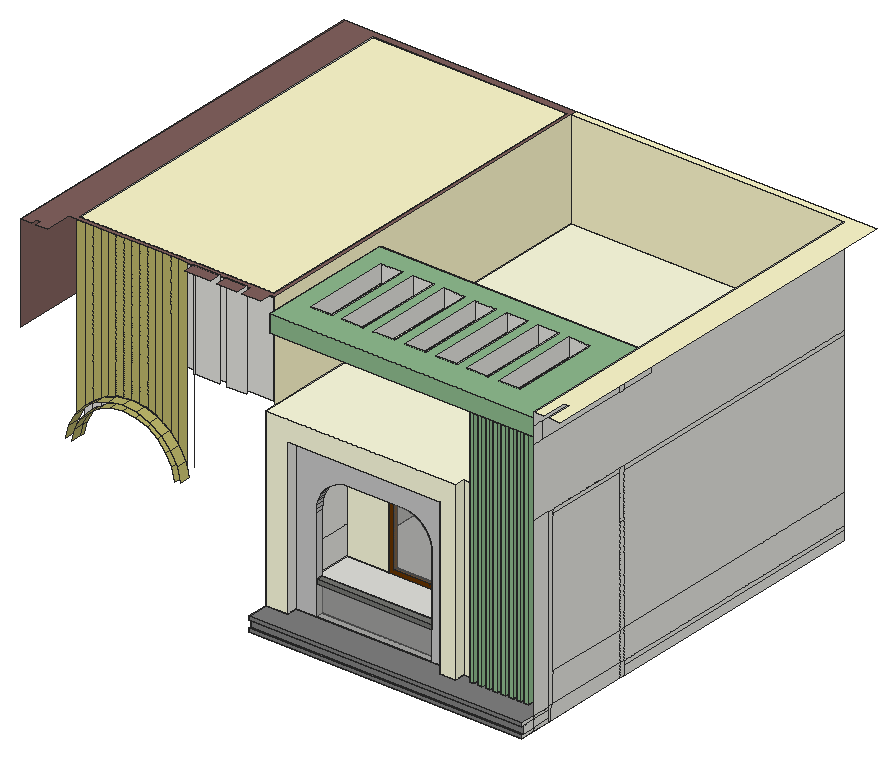
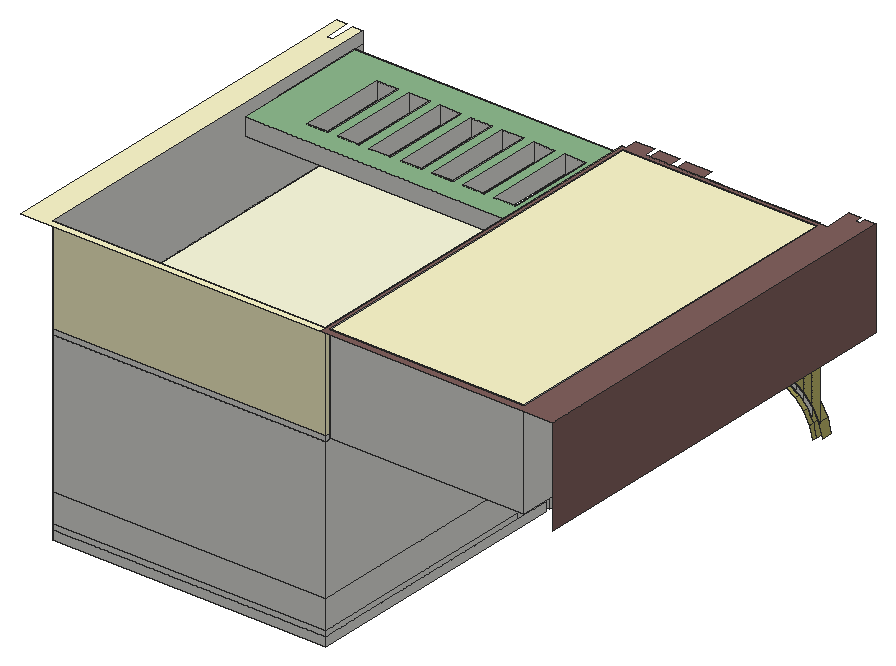
# SketchUp Ruby script. Lengths in inches.
U = 1.inch
M = Sketchup.active_model
def pt(a) = Geom::Point3d.new(a.map { |v| v * U })
def face(e, loops, mat)
  f = e.add_face(loops[0].map { |a| pt(a) })
  loops[1..].each { |l| e.add_face(l.map { |a| pt(a) }).erase! }
  f.material = f.back_material = mat if mat
  f
end
# faces: each face lists its corners as indices into pts; further lists are holes
def faces(e, pts, list, mat = nil) = list.each { |f| face(e, (f[0].is_a?(Array) ? f : [f]).map { |l| l.map { |i| pts[i] } }, mat) }
# xy, xz, yz: faces in a plane at the given z, y or x. An outline is a flat list of corners, or four numbers for a rectangle; further outlines are holes
def ring(l) = l.size == 4 ? [[l[0], l[1]], [l[2], l[1]], [l[2], l[3]], [l[0], l[3]]] : l.each_slice(2).to_a
def flat(e, list, mat, &to3) = list.each { |f| face(e, (f[0].is_a?(Array) ? f : [f]).map { |l| ring(l).map { |u, v| to3.(u, v) } }, mat) }
def xy(e, z, list, mat = nil) = flat(e, list, mat) { |x, y| [x, y, z] }
def xz(e, y, list, mat = nil) = flat(e, list, mat) { |x, z| [x, y, z] }
def yz(e, x, list, mat = nil) = flat(e, list, mat) { |y, z| [x, y, z] }
def lines(e, pts, list) = list.each { |a, b| e.add_line(pt(pts[a]), pt(pts[b])) }
# prism: a flat outline (further loops are holes) pulled along v
def prism(e, loops, v, mat = nil)
  f = face(e, loops, mat); d = Geom::Vector3d.new(v.map { |x| x * U })
  f.pushpull(f.normal.samedirection?(d) ? d.length : -d.length)
end
def box(e, o, s, mat = nil) = prism(e, [[o, [o[0] + s[0], o[1], o[2]], [o[0] + s[0], o[1] + s[1], o[2]], [o[0], o[1] + s[1], o[2]]]], [0, 0, s[2]], mat)
def at(x, y, z, deg = 0) = Geom::Transformation.translation(pt([x, y, z])) * Geom::Transformation.rotation(ORIGIN, Z_AXIS, deg.degrees)
def axes(o, x, y, z) = Geom::Transformation.new([*x, 0, *y, 0, *z, 0, *pt(o).to_a, 1])
def part(name) = M.definitions.add(name)
# library, detail: a bought-in or finely detailed component or shape, given as its bounding box
def library(name, o, s) = part(name).tap { |d| box(d.entities, o, s) }
def detail(e, o, s) = box(e.add_group.entities, o, s)
def put(e, d, t, mat = nil) = e.add_instance(d, t).tap { |i| i.material = mat if mat }
def group(e, t, mat = nil) = e.add_group.tap { |g| g.transformation = t; g.material = mat if mat }.entities
root = M.entities
M.materials.add("[0043_SaddleBrown]").color = [130, 97, 94]
M.materials.add("[0050_LemonChiffon]").color = [255, 250, 205]
M.materials.add("[0054_LightYellow]").color = [255, 255, 224]
M.materials.add("[0057_DarkKhaki]").color = [189, 183, 107]
M.materials.add("[0072_DarkSeaGreen]").color = [143, 188, 143]
M.materials.add("[0133_Gray]").color = [128, 128, 128]
M.materials.add("[Cladding Stucco White]").color = [200, 200, 200]
M.materials.add("[Color C08]").color = [102, 51, 0]
M.materials.add("[Color M00]").color = [255, 255, 255]
M.materials.add("[Metal Seamed]").color = [118, 119, 115]
M.materials.add("[Translucent Glass Gray]").color = [128, 128, 128]
M.materials["[Translucent Glass Gray]"].alpha = 0.5
M.materials.add("[Wood Floor Dark]").color = [153, 94, 42]
c1 = part("Group\#1")
xy(c1.entities,0,[[0,0,81.875,4.3125]],"[Color C08]")
xy(c1.entities,4.13,[[4.13,0,38.5,0.0625],[38.5,0,42.19,0.0625],[42.19,0,77.74,0.0625],[4.13,0.0625,38.5,4.3125],[38.5,0.0625,42.19,4.3125],
  [42.19,0.0625,77.74,4.3125]],"[Color C08]")
xy(c1.entities,128.34,[[4.13,0,38.5,0.0625],[42.19,0,77.74,0.0625],[4.13,0.0625,38.5,4.3125],[42.19,0.0625,77.74,4.3125]],"[Color C08]")
xy(c1.entities,132.48,[[0,0,81.875,4.3125]],"[Color C08]")
xz(c1.entities,0,[[[0,0,81.875,132.48],[4.13,4.13,4.13,128.34,38.5,128.34,38.5,4.13,42.19,4.13,42.19,128.34,77.74,128.34,77.74,4.13]]],"[Color C08]")
xz(c1.entities,0.0625,[[4.13,4.13,38.5,128.34],[42.19,4.13,77.74,128.34]],"[Translucent Glass Gray]")
xz(c1.entities,4.3125,[[[0,0,81.875,132.48],[4.13,4.13,77.74,4.13,77.74,128.34,42.19,128.34,42.19,4.13,38.5,4.13,38.5,128.34,4.13,128.34]]],"[Color C08]")
yz(c1.entities,0,[[0,0,4.3125,132.48]],"[Color C08]")
yz(c1.entities,4.13,[[0,4.13,0.0625,128.34],[0.0625,4.13,4.3125,128.34]],"[Color C08]")
yz(c1.entities,38.5,[[0,4.13,0.0625,128.34],[0.0625,4.13,4.3125,128.34]],"[Color C08]")
yz(c1.entities,42.19,[[0,4.13,0.0625,128.34],[0.0625,4.13,4.3125,128.34]],"[Color C08]")
yz(c1.entities,77.74,[[0,4.13,0.0625,128.34],[0.0625,4.13,4.3125,128.34]],"[Color C08]")
yz(c1.entities,81.875,[[0,0,4.3125,132.48]],"[Color C08]")
xy(root,302,[[287.625,134.125,287.625,173.6875,289.55,173.6875,289.55,167.4375,295.8,167.4375,295.8,173.6875,302.98,173.6875,302.98,167.4375,309.23,167.4375,309.23,173.6875,316.42,173.6875,316.42,167.4375,322.67,167.4375,322.67,173.6875,329.86,173.6875,329.86,167.4375,336.11,167.4375,336.11,173.6875,343.3,173.6875,343.3,167.4375,349.55,167.4375,349.55,173.6875,356.73,173.6875,356.73,167.4375,362.98,167.4375,362.98,173.6875,370.17,173.6875,370.17,167.4375,376.42,167.4375,376.42,173.6875,624.625,173.6875,624.625,134.125],[287.625,173.6875,624.625,285.75]],"[Wood Floor Dark]")
xy(root,306.0625,[[287.625,137,287.625,160.625,314.125,160.625,314.125,173.6875,502.3125,173.6875,502.3125,160.625,521.4375,160.625,521.4375,173.6875,534.24,173.6875,534.24,166.375,539.56,166.375,539.56,173.6875,544.06,173.6875,544.06,166.375,549.37,166.375,549.37,173.6875,553.87,173.6875,553.87,166.375,559.18,166.375,559.18,173.6875,563.68,173.6875,563.68,166.375,568.99,166.375,568.99,173.6875,573.49,173.6875,573.49,166.375,578.81,166.375,578.81,173.6875,583.31,173.6875,583.31,166.375,588.62,166.375,588.62,173.6875,592.87,173.6875,592.87,166.375,598.18,166.375,598.18,173.6875,601.68,173.6875,601.68,166.375,606.99,166.375,606.99,173.6875,624.625,173.6875,624.625,137]])
xy(root,306.0625,[[287.625,134.125,624.625,137]],"[0133_Gray]")
xy(root,313,[[287.625,291.75,624.625,631.8125]])
xy(root,315.1875,[[287.625,137,287.625,160.625,314.125,160.625,314.125,173.6875,502.3125,173.6875,502.3125,160.625,521.4375,160.625,521.4375,173.6875,534.24,173.6875,534.24,166.375,539.56,166.375,539.56,173.6875,544.06,173.6875,544.06,166.375,549.37,166.375,549.37,173.6875,553.87,173.6875,553.87,166.375,559.18,166.375,559.18,173.6875,563.68,173.6875,563.68,166.375,568.99,166.375,568.99,173.6875,573.49,173.6875,573.49,166.375,578.81,166.375,578.81,173.6875,583.31,173.6875,583.31,166.375,588.62,166.375,588.62,173.6875,592.87,173.6875,592.87,166.375,598.18,166.375,598.18,173.6875,601.68,173.6875,601.68,166.375,606.99,166.375,606.99,173.6875,624.625,173.6875,624.625,137]])
xy(root,315.1875,[[287.625,134.125,624.625,137]],"[0133_Gray]")
xy(root,319,[[287.625,160.625,314.125,173.6875],[502.3125,160.625,521.4375,173.6875],[534.24,166.375,539.56,173.6875],[544.06,166.375,549.37,173.6875],[553.87,166.375,559.18,173.6875],
  [563.68,166.375,568.99,173.6875],[573.49,166.375,578.81,173.6875],[583.31,166.375,588.62,173.6875],[592.87,166.375,598.18,173.6875],[601.68,166.375,606.99,173.6875],
  [287.625,173.6875,339.24,182.6875],[339.24,173.6875,481.81,182.6875],[287.625,182.6875,624.625,285.75],[287.625,291.75,624.625,631.8125]])
xy(root,319,[[287.625,134.125,624.625,134.125,624.625,173.6875,606.99,173.6875,606.99,166.375,601.68,166.375,601.68,173.6875,598.18,173.6875,598.18,166.375,592.87,166.375,592.87,173.6875,588.62,173.6875,588.62,166.375,583.31,166.375,583.31,173.6875,578.81,173.6875,578.81,166.375,573.49,166.375,573.49,173.6875,568.99,173.6875,568.99,166.375,563.68,166.375,563.68,173.6875,559.18,173.6875,559.18,166.375,553.87,166.375,553.87,173.6875,549.37,173.6875,549.37,166.375,544.06,166.375,544.06,173.6875,539.56,173.6875,539.56,166.375,534.24,166.375,534.24,173.6875,521.4375,173.6875,521.4375,160.625,502.3125,160.625,502.3125,173.6875,314.125,173.6875,314.125,160.625,287.625,160.625]],"[0133_Gray]")
xy(root,319,[[338.79,285.75,450.64,291.75]],"[Color M00]")
xy(root,355,[[339.24,173.6875,481.81,182.6875]],"[Metal Seamed]")
xy(root,360.5625,[[339.24,173.6875,481.81,182.6875]],"[Metal Seamed]")
xy(root,464.9,[[338.79,285.75,450.64,291.75]],"[Color M00]")
xy(root,476.93,[[370.28,173.6875,446.09,182.6875]],"[Cladding Stucco White]")
xy(root,509.25,[[314.125,160.625,502.3125,173.6875]],"[0050_LemonChiffon]")
xy(root,529,[[287.625,291.75,624.625,631.8125]])
xy(root,529,[[287.625,182.6875,624.625,285.75]],"[Wood Floor Dark]")
xy(root,535,[[287.625,160.625,521.4375,160.625,521.4375,173.6875,624.625,173.6875,624.625,631.8125,287.625,631.8125]],"[0054_LightYellow]")
xy(root,618.43,[[534.24,165.625,539.56,166.375],[544.06,165.625,549.37,166.375],[553.87,165.625,559.18,166.375],[563.68,165.625,568.99,166.375],[573.49,165.625,578.81,166.375],
  [583.31,165.625,588.62,166.375],[592.87,165.625,598.18,166.375],[601.68,165.625,606.99,166.375],[534.24,166.375,539.56,173.6875],[544.06,166.375,549.37,173.6875],
  [553.87,166.375,559.18,173.6875],[563.68,166.375,568.99,173.6875],[573.49,166.375,578.81,173.6875],[583.31,166.375,588.62,173.6875],[592.87,166.375,598.18,173.6875],
  [601.68,166.375,606.99,173.6875]])
xy(root,618.43,[[[287.625,165.625,287.625,335.55,624.625,335.55,624.625,165.625,606.99,165.625,606.99,173.6875,601.68,173.6875,601.68,165.625,598.18,165.625,598.18,173.6875,592.87,173.6875,592.87,165.625,588.62,165.625,588.62,173.6875,583.31,173.6875,583.31,165.625,578.81,165.625,578.81,173.6875,573.49,173.6875,573.49,165.625,568.99,165.625,568.99,173.6875,563.68,173.6875,563.68,165.625,559.18,165.625,559.18,173.6875,553.87,173.6875,553.87,165.625,549.37,165.625,549.37,173.6875,544.06,173.6875,544.06,165.625,539.56,165.625,539.56,173.6875,534.24,173.6875,534.24,165.625],[310.72,200.59,336.91,309.59],[349.35,200.59,375.54,309.59],[387.97,200.59,414.16,309.59],[426.6,200.59,452.79,309.59],[465.22,200.59,491.41,309.59],[503.85,200.59,530.04,309.59],[542.72,200.59,568.91,309.59]]],"[0072_DarkSeaGreen]")
xy(root,640.12,[[[287.625,165.625,624.625,335.55],[310.72,200.59,336.91,309.59],[349.35,200.59,375.54,309.59],[387.97,200.59,414.16,309.59],[426.6,200.59,452.79,309.59],[465.22,200.59,491.41,309.59],[503.85,200.59,530.04,309.59],[542.72,200.59,568.91,309.59]]],"[0072_DarkSeaGreen]")
xy(root,649,[[42.625,179.6875,282.1875,631.8125]])
xy(root,655,[[[0,140.625,14.17,140.625,14.17,148.6875,19.125,148.6875,19.125,140.625,33.625,140.625,33.625,173.6875,258.81,173.6875,258.81,159.3125,282.62,159.3125,282.62,173.6875,287.625,173.6875,287.625,640.8125,0,640.8125],[42.625,179.6875,282.1875,631.8125]],[187.68,159.3125,219.81,173.6875],[228.25,159.3125,252.93,173.6875]],"[0043_SaddleBrown]")
xy(root,655,[[624.625,152.625,637.14,152.625,637.14,183.8125,644.16,183.8125,644.16,152.625,657.3125,152.625,657.3125,640.8125,287.625,640.8125,287.625,631.8125,624.625,631.8125],[42.625,179.6875,282.1875,631.8125]],"[0050_LemonChiffon]")
xz(root,134.125,[[287.625,302,624.625,306.0625],[287.625,315.1875,624.625,319]],"[0133_Gray]")
xz(root,137,[[287.625,306.0625,624.625,315.1875]],"[0133_Gray]")
xz(root,160.625,[[287.625,306.0625,314.125,315.1875],[502.3125,306.0625,521.4375,315.1875],[287.625,315.1875,314.125,319],[502.3125,315.1875,521.4375,319]])
xz(root,160.625,[[287.625,319,314.125,319,314.125,509.25,502.3125,509.25,502.3125,319,521.4375,319,521.4375,535,287.625,535]],"[0054_LightYellow]")
xz(root,165.625,[[287.625,618.43,624.625,640.12]],"[0072_DarkSeaGreen]")
xz(root,166.375,[[534.24,306.0625,539.56,315.1875],[544.06,306.0625,549.37,315.1875],[553.87,306.0625,559.18,315.1875],[563.68,306.0625,568.99,315.1875],[573.49,306.0625,578.81,315.1875],
  [583.31,306.0625,588.62,315.1875],[592.87,306.0625,598.18,315.1875],[601.68,306.0625,606.99,315.1875],[534.24,315.1875,539.56,319],[544.06,315.1875,549.37,319],
  [553.87,315.1875,559.18,319],[563.68,315.1875,568.99,319],[573.49,315.1875,578.81,319],[583.31,315.1875,588.62,319],[592.87,315.1875,598.18,319],
  [601.68,315.1875,606.99,319]])
xz(root,166.375,[[534.24,319,539.56,618.43],[544.06,319,549.37,618.43],[553.87,319,559.18,618.43],[563.68,319,568.99,618.43],[573.49,319,578.81,618.43],
  [583.31,319,588.62,618.43],[592.87,319,598.18,618.43],[601.68,319,606.99,618.43]],"[0072_DarkSeaGreen]")
xz(root,173.6875,[[287.625,302,287.625,319,314.125,319,314.125,306.0625,502.3125,306.0625,502.3125,319,521.4375,319,521.4375,306.0625,534.24,306.0625,534.24,319,539.56,319,539.56,306.0625,544.06,306.0625,544.06,319,549.37,319,549.37,306.0625,553.87,306.0625,553.87,319,559.18,319,559.18,306.0625,563.68,306.0625,563.68,319,568.99,319,568.99,306.0625,573.49,306.0625,573.49,319,578.81,319,578.81,306.0625,583.31,306.0625,583.31,319,588.62,319,588.62,306.0625,592.87,306.0625,592.87,319,598.18,319,598.18,306.0625,601.68,306.0625,601.68,319,606.99,319,606.99,306.0625,624.625,306.0625,624.625,302],[314.125,306.0625,339.24,315.1875],[339.24,306.0625,481.81,315.1875],[481.81,306.0625,502.3125,315.1875],[521.4375,306.0625,534.24,315.1875],
  [539.56,306.0625,544.06,315.1875],[549.37,306.0625,553.87,315.1875],[559.18,306.0625,563.68,315.1875],[568.99,306.0625,573.49,315.1875],[578.81,306.0625,583.31,315.1875],
  [588.62,306.0625,592.87,315.1875],[598.18,306.0625,601.68,315.1875],[606.99,306.0625,624.625,315.1875],[314.125,315.1875,339.24,319],[339.24,315.1875,481.81,319],
  [481.81,315.1875,502.3125,319],[521.4375,315.1875,534.24,319],[539.56,315.1875,544.06,319],[549.37,315.1875,553.87,319],[559.18,315.1875,563.68,319],
  [568.99,315.1875,573.49,319],[578.81,315.1875,583.31,319],[588.62,315.1875,592.87,319],[598.18,315.1875,601.68,319],[606.99,315.1875,624.625,319],
  [534.24,319,539.56,535],[544.06,319,549.37,535],[553.87,319,559.18,535],[563.68,319,568.99,535],[573.49,319,578.81,535],
  [583.31,319,588.62,535],[592.87,319,598.18,535],[601.68,319,606.99,535],[169.4375,434.51,163.875,444.68,159.75,449.21,159.75,459.71,169.4375,449.07],[53.1875,435.52,53.1875,449.68,62.875,460.32,62.875,449.8125,58.2,444.68],
  [159.75,449.21,153.51,456.0625,150.0625,458.39,150.0625,466.93,158.17,461.45,159.75,459.71],[62.875,449.8125,62.875,460.32,63.9,461.45,72.5625,467.3,72.5625,458.77,68.5625,456.0625],[150.0625,458.39,140.75,464.6875,140.375,464.83,140.375,472.375,144.02,471.02,150.0625,466.93],[72.5625,458.77,72.5625,467.3,78.06,471.02,82.25,472.58,82.25,465.03,81.32,464.6875],[140.375,464.83,130.6875,468.4375,130.6875,475.98,140.375,472.375],
  [82.25,465.03,82.25,472.58,91.9375,476.1875,91.9375,468.64],[130.6875,468.4375,126.33,470.0625,121,470.7,121,477.82,128,476.98,130.6875,475.98],[91.9375,468.64,91.9375,476.1875,94.07,476.98,101.625,477.89,101.625,470.76,95.75,470.0625],[121,470.7,111.3125,471.86,111.3125,478.98,121,477.82],[101.625,470.76,101.625,477.89,111.04,479.01,111.3125,478.98,111.3125,471.86,111.04,471.89],
  [187.68,535,188.8125,655],[188.8125,535,219.81,655],[228.25,535,252.93,655],[534.24,535,539.56,618.43],[544.06,535,549.37,618.43],
  [553.87,535,559.18,618.43],[563.68,535,568.99,618.43],[573.49,535,578.81,618.43],[583.31,535,588.62,618.43],[592.87,535,598.18,618.43],
  [601.68,535,606.99,618.43]])
xz(root,173.6875,[[521.4375,319,534.24,535],[539.56,319,544.06,535],[549.37,319,553.87,535],[559.18,319,563.68,535],[568.99,319,573.49,535],
  [578.81,319,583.31,535],[588.62,319,592.87,535],[598.18,319,601.68,535],[606.99,319,624.625,535]],"[0054_LightYellow]")
xz(root,173.6875,[[179.125,429.18,179.125,655,169.4375,655,169.4375,449.07,169.67,448.8125,177.88,433.82],[43.5,431.23,44.2,433.82,52.4,448.8125,53.1875,449.68,53.1875,655,43.5,655],[169.4375,449.07,169.4375,655,159.75,655,159.75,459.71],[53.1875,449.68,62.875,460.32,62.875,655,53.1875,655],[159.75,459.71,159.75,655,150.0625,655,150.0625,466.93,158.17,461.45],
  [62.875,460.32,63.9,461.45,72.5625,467.3,72.5625,655,62.875,655],[150.0625,466.93,150.0625,655,140.375,655,140.375,472.375,144.02,471.02],[72.5625,467.3,78.06,471.02,82.25,472.58,82.25,655,72.5625,655],[140.375,472.375,140.375,655,130.6875,655,130.6875,475.98],[82.25,472.58,91.9375,476.1875,91.9375,655,82.25,655],
  [130.6875,475.98,130.6875,655,121,655,121,477.82,128,476.98],[91.9375,476.1875,94.07,476.98,101.625,477.89,101.625,655,91.9375,655],[121,477.82,121,655,111.3125,655,111.3125,478.98],[101.625,477.89,111.04,479.01,111.3125,478.98,111.3125,655,101.625,655]],"[0057_DarkKhaki]")
xz(root,173.6875,[[314.125,319,339.24,319,339.24,434.32,339.49,439.01,340.22,443.65,341.4375,448.18,343.125,452.5625,345.26,456.75,347.82,460.68,350.78,464.32,354.11,467.64,357.76,470.59,361.7,473.14,365.89,475.26,370.28,476.93,446.09,476.93,450.75,476.625,455.33,475.71,459.76,474.21,463.95,472.15,467.83,469.55,471.35,466.47,474.43,462.96,477.02,459.07,479.09,454.88,480.59,450.46,481.5,445.875,481.81,441.21,481.81,319,502.3125,319,502.3125,509.25,314.125,509.25]],"[Cladding Stucco White]")
xz(root,173.6875,[[339.24,355,481.81,360.5625]],"[Metal Seamed]")
xz(root,173.6875,[[339.24,319,481.81,355]],"[Translucent Glass Gray]")
xz(root,179.6875,[[42.625,535,282.1875,649],[42.625,649,282.1875,655]])
xz(root,182.6875,[[287.625,319,339.24,355],[481.81,319,481.81,441.21,481.5,445.875,480.59,450.46,479.09,454.88,477.02,459.07,474.43,462.96,471.35,466.47,467.83,469.55,463.95,472.15,459.76,474.21,455.33,475.71,450.75,476.625,446.09,476.93,370.28,476.93,365.89,475.26,361.7,473.14,357.76,470.59,354.11,467.64,350.78,464.32,347.82,460.68,345.26,456.75,343.125,452.5625,341.4375,448.18,340.22,443.65,339.49,439.01,339.24,434.32,339.24,355,287.625,355,287.625,529,624.625,529,624.625,319]])
xz(root,182.6875,[[339.24,355,481.81,360.5625]],"[Metal Seamed]")
xz(root,182.6875,[[339.24,319,481.81,355]],"[Translucent Glass Gray]")
xz(root,200.59,[[310.72,618.43,336.91,640.12],[349.35,618.43,375.54,640.12],[387.97,618.43,414.16,640.12],[426.6,618.43,452.79,640.12],[465.22,618.43,491.41,640.12],
  [503.85,618.43,530.04,640.12],[542.72,618.43,568.91,640.12]])
xz(root,285.75,[[287.625,302,624.625,319]])
xz(root,285.75,[[287.625,319,287.625,529,624.625,529,624.625,319,450.64,319,450.64,464.9,338.79,464.9,338.79,319]],"[0054_LightYellow]")
xz(root,291.75,[[287.625,302,624.625,313],[287.625,313,338.79,319],[338.79,313,450.64,319],[450.64,313,624.625,319],[287.625,319,287.625,529,624.625,529,624.625,319,450.64,319,450.64,464.9,338.79,464.9,338.79,319]])
xz(root,309.59,[[310.72,618.43,336.91,640.12],[349.35,618.43,375.54,640.12],[387.97,618.43,414.16,640.12],[426.6,618.43,452.79,640.12],[465.22,618.43,491.41,640.12],
  [503.85,618.43,530.04,640.12],[542.72,618.43,568.91,640.12]])
xz(root,335.55,[[287.625,618.43,624.625,640.12]])
xz(root,631.8125,[[287.625,302,624.625,313],[287.625,313,624.625,319],[287.625,319,624.625,355],[287.625,355,624.625,529],[287.625,529,624.625,535],
  [42.625,535,282.1875,649],[42.625,649,282.1875,655]])
xz(root,631.8125,[[287.625,535,624.625,655]],"[0050_LemonChiffon]")
yz(root,0,[[140.625,535,640.8125,655]],"[0043_SaddleBrown]")
yz(root,42.625,[[179.6875,535,631.8125,649],[179.6875,649,188.6875,655],[188.6875,649,631.8125,655]])
yz(root,282.1875,[[179.6875,535,631.8125,649],[179.6875,649,631.8125,655]])
yz(root,287.625,[[173.6875,302,179.6875,319],[179.6875,302,285.75,319],[291.75,302,631.8125,313],[291.75,313,311.4,319],[311.4,313,336.53,319],
  [336.53,313,631.8125,319],[160.625,319,173.6875,355],[173.6875,319,182.6875,355],[182.6875,319,285.75,355],[291.75,319,631.8125,355],
  [160.625,355,173.6875,535],[173.6875,355,182.6875,535],[182.6875,355,285.75,529],[291.75,355,631.8125,529],[182.6875,529,234.22,535],
  [234.22,529,285.75,535],[291.75,529,307.19,535],[307.19,529,353.82,535],[353.82,529,631.8125,535],[165.625,618.43,173.6875,640.12],
  [173.6875,618.43,335.55,640.12]])
yz(root,287.625,[[173.6875,535,631.8125,535,631.8125,655,173.6875,655,173.6875,640.12,335.55,640.12,335.55,618.43,173.6875,618.43]],"[0050_LemonChiffon]")
yz(root,287.625,[[134.125,302,134.125,306.0625,160.625,306.0625,160.625,319,173.6875,319,173.6875,302],[137,306.0625,160.625,315.1875],[134.125,315.1875,160.625,319]],"[0133_Gray]")
yz(root,310.72,[[200.59,618.43,309.59,640.12]])
yz(root,314.125,[[160.625,306.0625,173.6875,315.1875],[160.625,315.1875,173.6875,319],[160.625,319,173.6875,509.25]])
yz(root,336.91,[[200.59,618.43,309.59,640.12]])
yz(root,338.79,[[285.75,319,291.75,464.9]],"[Color M00]")
yz(root,339.24,[[173.6875,319,182.6875,355]])
yz(root,339.24,[[173.6875,360.5625,182.6875,434.32]],"[Cladding Stucco White]")
yz(root,339.24,[[173.6875,355,182.6875,360.5625]],"[Metal Seamed]")
yz(root,349.35,[[200.59,618.43,309.59,640.12]])
yz(root,375.54,[[200.59,618.43,309.59,640.12]])
yz(root,387.97,[[200.59,618.43,309.59,640.12]])
yz(root,414.16,[[200.59,618.43,309.59,640.12]])
yz(root,426.6,[[200.59,618.43,309.59,640.12]])
yz(root,450.64,[[285.75,319,291.75,464.9]],"[Color M00]")
yz(root,452.79,[[200.59,618.43,309.59,640.12]])
yz(root,465.22,[[200.59,618.43,309.59,640.12]])
yz(root,481.81,[[173.6875,360.5625,182.6875,441.21]],"[Cladding Stucco White]")
yz(root,481.81,[[173.6875,355,182.6875,360.5625]],"[Metal Seamed]")
yz(root,491.41,[[200.59,618.43,309.59,640.12]])
yz(root,502.3125,[[160.625,306.0625,173.6875,315.1875],[160.625,315.1875,173.6875,319],[160.625,319,173.6875,509.25]])
yz(root,503.85,[[200.59,618.43,309.59,640.12]])
yz(root,521.4375,[[160.625,306.0625,173.6875,315.1875],[160.625,315.1875,173.6875,319]])
yz(root,521.4375,[[160.625,319,173.6875,535]],"[0054_LightYellow]")
yz(root,530.04,[[200.59,618.43,309.59,640.12]])
yz(root,534.24,[[166.375,306.0625,173.6875,315.1875],[166.375,315.1875,173.6875,319]])
yz(root,534.24,[[166.375,319,173.6875,618.43]],"[0072_DarkSeaGreen]")
yz(root,539.56,[[166.375,306.0625,173.6875,315.1875],[166.375,315.1875,173.6875,319]])
yz(root,539.56,[[166.375,319,173.6875,618.43]],"[0072_DarkSeaGreen]")
yz(root,542.72,[[200.59,618.43,309.59,640.12]])
yz(root,544.06,[[166.375,306.0625,173.6875,315.1875],[166.375,315.1875,173.6875,319]])
yz(root,544.06,[[166.375,319,173.6875,618.43]],"[0072_DarkSeaGreen]")
yz(root,549.37,[[166.375,306.0625,173.6875,315.1875],[166.375,315.1875,173.6875,319]])
yz(root,549.37,[[166.375,319,173.6875,618.43]],"[0072_DarkSeaGreen]")
yz(root,553.87,[[166.375,306.0625,173.6875,315.1875],[166.375,315.1875,173.6875,319]])
yz(root,553.87,[[166.375,319,173.6875,618.43]],"[0072_DarkSeaGreen]")
yz(root,559.18,[[166.375,306.0625,173.6875,315.1875],[166.375,315.1875,173.6875,319]])
yz(root,559.18,[[166.375,319,173.6875,618.43]],"[0072_DarkSeaGreen]")
yz(root,563.68,[[166.375,306.0625,173.6875,315.1875],[166.375,315.1875,173.6875,319]])
yz(root,563.68,[[166.375,319,173.6875,618.43]],"[0072_DarkSeaGreen]")
yz(root,568.91,[[200.59,618.43,309.59,640.12]])
yz(root,568.99,[[166.375,306.0625,173.6875,315.1875],[166.375,315.1875,173.6875,319]])
yz(root,568.99,[[166.375,319,173.6875,618.43]],"[0072_DarkSeaGreen]")
yz(root,573.49,[[166.375,306.0625,173.6875,315.1875],[166.375,315.1875,173.6875,319]])
yz(root,573.49,[[166.375,319,173.6875,618.43]],"[0072_DarkSeaGreen]")
yz(root,578.81,[[166.375,306.0625,173.6875,315.1875],[166.375,315.1875,173.6875,319]])
yz(root,578.81,[[166.375,319,173.6875,618.43]],"[0072_DarkSeaGreen]")
yz(root,583.31,[[166.375,306.0625,173.6875,315.1875],[166.375,315.1875,173.6875,319]])
yz(root,583.31,[[166.375,319,173.6875,618.43]],"[0072_DarkSeaGreen]")
yz(root,588.62,[[166.375,306.0625,173.6875,315.1875],[166.375,315.1875,173.6875,319]])
yz(root,588.62,[[166.375,319,173.6875,618.43]],"[0072_DarkSeaGreen]")
yz(root,592.87,[[166.375,306.0625,173.6875,315.1875],[166.375,315.1875,173.6875,319]])
yz(root,592.87,[[166.375,319,173.6875,618.43]],"[0072_DarkSeaGreen]")
yz(root,598.18,[[166.375,306.0625,173.6875,315.1875],[166.375,315.1875,173.6875,319]])
yz(root,598.18,[[166.375,319,173.6875,618.43]],"[0072_DarkSeaGreen]")
yz(root,601.68,[[166.375,306.0625,173.6875,315.1875],[166.375,315.1875,173.6875,319]])
yz(root,601.68,[[166.375,319,173.6875,618.43]],"[0072_DarkSeaGreen]")
yz(root,606.99,[[166.375,306.0625,173.6875,315.1875],[166.375,315.1875,173.6875,319]])
yz(root,606.99,[[166.375,319,173.6875,618.43]],"[0072_DarkSeaGreen]")
yz(root,624.625,[[134.125,302,152.625,306.0625],[152.625,302,173.6875,306.0625],[173.6875,302,179.6875,319],[179.6875,302,285.75,319],[285.75,302,291.75,319],
  [291.75,302,631.8125,313],[137,306.0625,152.625,315.1875],[152.625,306.0625,173.6875,315.1875],[291.75,313,631.8125,319],[134.125,315.1875,152.625,319],
  [152.625,315.1875,173.6875,319],[152.625,319,173.6875,535],[173.6875,319,182.6875,535],[182.6875,319,285.75,355],[285.75,319,291.75,355],
  [291.75,319,631.8125,355],[182.6875,355,285.75,529],[285.75,355,291.75,475],[291.75,355,631.8125,529],[285.75,475,291.75,535],
  [182.6875,529,285.75,535],[291.75,529,631.8125,535],[152.625,535,152.625,618.43,335.55,618.43,335.55,640.12,152.625,640.12,152.625,655,631.8125,655,631.8125,535],[152.625,618.43,165.625,640.12],[165.625,618.43,285.75,640.12],
  [285.75,618.43,291.75,640.12],[291.75,618.43,335.55,640.12]])
p = [[46.83,173.6875,416.39],[50.81,173.6875,431.17],[50.81,160.875,431.17],[46.83,160.875,416.39],[171.27,173.6875,431.17],[175.25,173.6875,416.39],
  [175.25,160.875,416.39],[171.27,160.875,431.17],[46.83,179.6875,416.39],[50.81,179.6875,431.17],[171.27,179.6875,431.17],[175.25,179.6875,416.39],
  [43.5,173.6875,431.23],[39.76,173.6875,417.32],[39.76,160.875,417.32],[44.2,160.875,433.82],[44.2,173.6875,433.82],[179.125,173.6875,429.18],
  [177.88,173.6875,433.82],[177.88,160.875,433.82],[182.32,160.875,417.32],[182.32,173.6875,417.32],[53.1875,173.6875,435.52],[58.2,173.6875,444.68],
  [58.2,160.875,444.68],[169.4375,173.6875,434.51],[163.875,160.875,444.68],[163.875,173.6875,444.68],[58.2,179.6875,444.68],[163.875,179.6875,444.68],
  [52.4,173.6875,448.8125],[52.4,160.875,448.8125],[169.67,173.6875,448.8125],[169.67,160.875,448.8125],[339.49,173.6875,439.01],[339.24,173.6875,434.32],
  [339.24,182.6875,434.32],[339.49,182.6875,439.01],[340.22,173.6875,443.65],[340.22,182.6875,443.65],[481.81,173.6875,441.21],[481.5,173.6875,445.875],
  [481.5,182.6875,445.875],[481.81,182.6875,441.21],[341.4375,173.6875,448.18],[341.4375,182.6875,448.18],[62.875,173.6875,449.8125],[68.5625,173.6875,456.0625],
  [68.5625,160.875,456.0625],[159.75,173.6875,449.21],[153.51,160.875,456.0625],[153.51,173.6875,456.0625],[68.5625,179.6875,456.0625],[153.51,179.6875,456.0625],
  [480.59,173.6875,450.46],[480.59,182.6875,450.46],[343.125,173.6875,452.5625],[343.125,182.6875,452.5625],[53.1875,173.6875,449.68],[63.9,160.875,461.45],
  [63.9,173.6875,461.45],[62.875,173.6875,460.32],[159.75,173.6875,459.71],[158.17,173.6875,461.45],[158.17,160.875,461.45],[169.4375,173.6875,449.07],
  [479.09,173.6875,454.88],[479.09,182.6875,454.88],[345.26,173.6875,456.75],[345.26,182.6875,456.75],[477.02,173.6875,459.07],[477.02,182.6875,459.07],
  [72.5625,173.6875,458.77],[81.32,173.6875,464.6875],[81.32,160.875,464.6875],[150.0625,173.6875,458.39],[140.75,160.875,464.6875],[140.75,173.6875,464.6875],
  [81.32,179.6875,464.6875],[140.75,179.6875,464.6875],[347.82,173.6875,460.68],[347.82,182.6875,460.68],[474.43,173.6875,462.96],[474.43,182.6875,462.96],
  [350.78,173.6875,464.32],[350.78,182.6875,464.32],[72.5625,173.6875,467.3],[78.06,160.875,471.02],[78.06,173.6875,471.02],[150.0625,173.6875,466.93],
  [144.02,173.6875,471.02],[144.02,160.875,471.02],[471.35,173.6875,466.47],[471.35,182.6875,466.47],[354.11,173.6875,467.64],[354.11,182.6875,467.64],
  [91.9375,173.6875,468.64],[95.75,173.6875,470.0625],[95.75,160.875,470.0625],[82.25,173.6875,465.03],[140.375,173.6875,464.83],[126.33,160.875,470.0625],
  [126.33,173.6875,470.0625],[130.6875,173.6875,468.4375],[95.75,179.6875,470.0625],[126.33,179.6875,470.0625],[467.83,173.6875,469.55],[467.83,182.6875,469.55],
  [357.76,173.6875,470.59],[357.76,182.6875,470.59],[463.95,173.6875,472.15],[463.95,182.6875,472.15],[101.625,173.6875,470.76],[111.04,173.6875,471.89],
  [111.04,160.875,471.89],[121,173.6875,470.7],[111.3125,173.6875,471.86],[99.41,179.6875,470.5],[111.04,179.6875,471.89],[361.7,173.6875,473.14],
  [361.7,182.6875,473.14],[82.25,173.6875,472.58],[94.07,160.875,476.98],[94.07,173.6875,476.98],[91.9375,173.6875,476.1875],[130.6875,173.6875,475.98],
  [128,173.6875,476.98],[128,160.875,476.98],[140.375,173.6875,472.375],[459.76,173.6875,474.21],[459.76,182.6875,474.21],[365.89,173.6875,475.26],
  [365.89,182.6875,475.26],[455.33,173.6875,475.71],[455.33,182.6875,475.71],[370.28,173.6875,476.93],[370.28,182.6875,476.93],[450.75,173.6875,476.625],
  [450.75,182.6875,476.625],[446.09,173.6875,476.93],[446.09,182.6875,476.93],[101.625,173.6875,477.89],[111.04,160.875,479.01],[111.04,173.6875,479.01],
  [111.3125,173.6875,478.98],[121,173.6875,477.82],[314.125,173.6875,355],[287.625,173.6875,355],[188.8125,173.6875,535],[188.8125,173.6875,431.23]]
faces(root,p,[[0,1,2,3],[4,5,6,7],[1,0,8,9],[5,4,10,11],[12,13,14,15,16],[17,18,19,20,21],[22,23,24,2,1],[25,4,7,26,27],
  [23,22,1,9,28],[4,25,27,29,10],[30,16,15,31],[18,32,33,19],[46,47,48,24,23],[49,27,26,50,51],[47,46,23,28,52],[27,49,51,53,29],
  [58,30,31,59,60,61],[62,63,64,33,32,65],[72,73,74,48,47],[75,51,50,76,77],[73,72,47,52,78],[51,75,77,79,53],[86,60,59,87,88],[89,90,91,64,63],
  [96,97,98,74,73,99],[100,77,76,101,102,103],[97,96,99,73,78,104],[77,100,103,102,105,79],[112,113,114,98,97],[115,102,101,114,113,116],[113,112,97,104,117,118],[102,115,116,113,118,105],
  [121,88,87,122,123,124],[125,126,127,91,90,128],[141,123,122,142,143],[144,143,142,127,126,145]],"[0057_DarkKhaki]")
faces(root,p,[[34,35,36,37],[38,34,37,39],[40,41,42,43],[44,38,39,45],[41,54,55,42],[56,44,45,57],[54,66,67,55],[68,56,57,69],
  [66,70,71,67],[80,68,69,81],[70,82,83,71],[84,80,81,85],[82,92,93,83],[94,84,85,95],[92,106,107,93],[108,94,95,109],
  [106,110,111,107],[119,108,109,120],[110,129,130,111],[131,119,120,132],[129,133,134,130],[135,131,132,136],[133,137,138,134],[137,139,140,138]],"[Cladding Stucco White]")
lines(root,p,[[146,147],[148,149]])
put(root,c1,axes([339.53,285.75,319],[1.35715,0,0],[0,1.155,0],[0,0,1.10136]))
